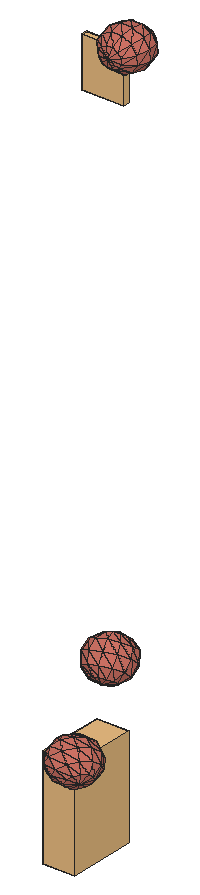
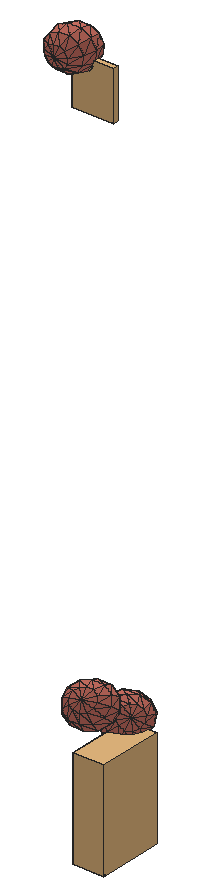
# SketchUp Ruby script. Lengths in inches.
U = 1.inch
M = Sketchup.active_model
def pt(a) = Geom::Point3d.new(a.map { |v| v * U })
def face(e, loops, mat)
  f = e.add_face(loops[0].map { |a| pt(a) })
  loops[1..].each { |l| e.add_face(l.map { |a| pt(a) }).erase! }
  f.material = f.back_material = mat if mat
  f
end
# faces: each face lists its corners as indices into pts; further lists are holes
def faces(e, pts, list, mat = nil) = list.each { |f| face(e, (f[0].is_a?(Array) ? f : [f]).map { |l| l.map { |i| pts[i] } }, mat) }
# xy, xz, yz: faces in a plane at the given z, y or x. An outline is a flat list of corners, or four numbers for a rectangle; further outlines are holes
def ring(l) = l.size == 4 ? [[l[0], l[1]], [l[2], l[1]], [l[2], l[3]], [l[0], l[3]]] : l.each_slice(2).to_a
def flat(e, list, mat, &to3) = list.each { |f| face(e, (f[0].is_a?(Array) ? f : [f]).map { |l| ring(l).map { |u, v| to3.(u, v) } }, mat) }
def xy(e, z, list, mat = nil) = flat(e, list, mat) { |x, y| [x, y, z] }
def xz(e, y, list, mat = nil) = flat(e, list, mat) { |x, z| [x, y, z] }
def yz(e, x, list, mat = nil) = flat(e, list, mat) { |y, z| [x, y, z] }
def lines(e, pts, list) = list.each { |a, b| e.add_line(pt(pts[a]), pt(pts[b])) }
# prism: a flat outline (further loops are holes) pulled along v
def prism(e, loops, v, mat = nil)
  f = face(e, loops, mat); d = Geom::Vector3d.new(v.map { |x| x * U })
  f.pushpull(f.normal.samedirection?(d) ? d.length : -d.length)
end
def box(e, o, s, mat = nil) = prism(e, [[o, [o[0] + s[0], o[1], o[2]], [o[0] + s[0], o[1] + s[1], o[2]], [o[0], o[1] + s[1], o[2]]]], [0, 0, s[2]], mat)
def at(x, y, z, deg = 0) = Geom::Transformation.translation(pt([x, y, z])) * Geom::Transformation.rotation(ORIGIN, Z_AXIS, deg.degrees)
def axes(o, x, y, z) = Geom::Transformation.new([*x, 0, *y, 0, *z, 0, *pt(o).to_a, 1])
def part(name) = M.definitions.add(name)
# library, detail: a bought-in or finely detailed component or shape, given as its bounding box
def library(name, o, s) = part(name).tap { |d| box(d.entities, o, s) }
def detail(e, o, s) = box(e.add_group.entities, o, s)
def put(e, d, t, mat = nil) = e.add_instance(d, t).tap { |i| i.material = mat if mat }
def group(e, t, mat = nil) = e.add_group.tap { |g| g.transformation = t; g.material = mat if mat }.entities
root = M.entities
M.materials.add("green").color = [174, 139, 102]
M.materials.add("vio").color = [206, 114, 100]
c1 = part("3DGeom~239_Defintion")
p = [[90.53,-63.37,-491.99],[67.74,-328.31,-318.83],[-81.52,-183.54,-449.92],[266.4,-189.55,-367.41],[200.76,100.79,-448.8],[-109.61,79.79,-484.74],
  [-45.97,174.5625,-459.8],[-208.9375,10.41,-460.45],[-280.37,201.57,-347.6],[-269.29,-227.52,-333.86],[-317.35,-14.98,-393.44],[-35.07,269.34,-392.33],
  [-149.08,-379.1,-184.82],[393.68,0,-317.54],[219.63,264.9375,-331.92],[-317.35,-14.98,-393.44],[-269.29,-227.52,-333.86],[-422.46,-183.54,-174.92],
  [-317.35,-14.98,-393.44],[-405.78,10.41,-301.68],[-405.78,10.41,-301.68],[-79.84,338.72,-300.39],[-79.84,338.72,-300.39],[219.63,264.9375,-331.92],
  [-35.07,269.34,-392.33],[266.4,-189.55,-367.41],[198.85,-385.11,-102.31],[67.74,-328.31,-318.83],[266.4,-189.55,-367.41],[370.9,-264.9375,-144.38],
  [393.68,0,-317.54],[370.9,-264.9375,-144.38],[266.4,-189.55,-367.41],[-450.55,79.79,-209.74],[-280.37,201.57,-347.6],[-439.65,174.5625,-142.26],
  [-280.37,201.57,-347.6],[-376.01,269.34,-117.33],[-280.37,201.57,-347.6],[-276.68,338.72,-141.62],[-280.37,201.57,-347.6],[-168.27,364.11,-208.62],
  [-276.68,338.72,-141.62],[-168.27,364.11,-208.62],[-280.37,201.57,-347.6],[-269.29,-227.52,-333.86],[-149.08,-379.1,-184.82],[-325.95,-328.31,-1.29],
  [-269.29,-227.52,-333.86],[415.48,189.55,-182.59],[142.09,385.11,-172.68],[415.48,189.55,-182.59],[219.63,264.9375,-331.92],[-79.84,338.72,-300.39],
  [219.63,264.9375,-331.92],[67.74,-328.31,-318.83],[11.08,-429.09,13.74],[-149.08,-379.1,-184.82],[67.74,-328.31,-318.83],[393.68,0,-317.54],
  [481.125,-100.79,-101.2],[370.9,-264.9375,-144.38],[415.48,189.55,-182.59],[393.68,0,-317.54],[-500,-63.37,-15.68],[-168.27,364.11,-208.62],
  [-79.84,338.72,-300.39],[-481.125,100.79,101.2],[-11.08,429.09,-13.74],[-168.27,364.11,-208.62],[-168.27,364.11,-208.62],[-149.08,-379.1,-184.82],
  [-142.09,-385.11,172.68],[-149.08,-379.1,-184.82],[-325.95,-328.31,-1.29],[415.48,189.55,-182.59],[500,63.37,15.68],[325.95,328.31,1.29],
  [415.48,189.55,-182.59],[325.95,328.31,1.29],[415.48,189.55,-182.59],[-415.48,-189.55,182.59],[276.68,-338.72,141.62],[376.01,-269.34,117.33],
  [376.01,-269.34,117.33],[370.9,-264.9375,-144.38],[-370.9,264.9375,144.38],[-370.9,264.9375,144.38],[-376.01,269.34,-117.33],[-198.85,385.11,102.31],
  [-376.01,269.34,-117.33],[-370.9,264.9375,144.38],[168.27,-364.11,208.62],[439.65,-174.5625,142.26],[376.01,-269.34,117.33],[-393.68,0,317.54],
  [149.08,379.1,184.82],[-325.95,-328.31,-1.29],[-219.63,-264.9375,331.93],[-325.95,-328.31,-1.29],[-219.63,-264.9375,331.93],[-415.48,-189.55,182.59],
  [325.95,328.31,1.29],[422.46,183.54,174.92],[149.08,379.1,184.82],[325.95,328.31,1.29],[79.84,-338.72,300.39],[450.55,-79.79,209.74],
  [-266.4,189.55,367.41],[-266.4,189.55,367.41],[-370.9,264.9375,144.38],[-67.74,328.31,318.83],[276.68,-338.72,141.62],[376.01,-269.34,117.33],
  [280.37,-201.57,347.6],[376.01,-269.34,117.33],[280.37,-201.57,347.6],[280.37,-201.57,347.6],[280.37,-201.57,347.6],[-266.4,189.55,367.41],
  [35.07,-269.34,392.33],[-219.63,-264.9375,331.93],[35.07,-269.34,392.33],[405.78,-10.41,301.68],[269.29,227.52,333.86],[149.08,379.1,184.82],
  [-415.48,-189.55,182.59],[-219.63,-264.9375,331.93],[-200.76,-100.78,448.8],[-415.48,-189.55,182.59],[-393.68,0,317.54],[-67.74,328.31,318.83],
  [269.29,227.52,333.86],[149.08,379.1,184.82],[79.84,-338.72,300.39],[168.27,-364.11,208.62],[280.37,-201.57,347.6],[280.37,-201.57,347.6],
  [35.07,-269.34,392.33],[79.84,-338.72,300.39],[280.37,-201.57,347.6],[405.78,-10.41,301.68],[317.35,14.98,393.44],[280.37,-201.57,347.6],
  [317.35,14.98,393.44],[-393.68,0,317.54],[-90.53,63.37,491.99],[-393.68,0,317.54],[-266.4,189.55,367.41],[-266.4,189.55,367.41],
  [81.52,183.54,449.92],[-67.74,328.31,318.83],[-67.74,328.31,318.83],[269.29,227.52,333.86],[45.97,-174.5625,459.8],[317.35,14.98,393.44],
  [269.29,227.52,333.86],[280.37,-201.57,347.6],[109.61,-79.79,484.74],[280.37,-201.57,347.6],[208.9375,-10.41,460.45],[280.37,-201.57,347.6],
  [317.35,14.98,393.44],[280.37,-201.57,347.6],[-266.4,189.55,367.41],[317.35,14.98,393.44]]
faces(c1.entities,p,[[0,1,2],[0,3,1],[4,3,0],[5,0,2],[6,0,5],[6,4,0],[5,2,7],[5,7,8],
  [6,5,8],[7,9,10],[7,2,9],[7,10,8],[11,4,6],[11,6,8],[2,12,9],[2,1,12],
  [4,13,3],[14,13,4],[11,14,4],[15,16,17],[18,17,19],[10,20,8],[21,11,8],[22,23,24],
  [25,26,27],[28,29,26],[30,31,32],[19,33,34],[33,35,36],[35,37,38],[37,39,40],[41,21,8],
  [42,43,44],[45,46,47],[48,47,17],[14,49,13],[50,51,52],[53,50,54],[55,56,57],[58,26,56],
  [59,60,61],[62,60,63],[19,17,64],[19,64,33],[65,50,66],[33,64,67],[33,67,35],[42,68,69],
  [70,68,50],[71,56,72],[73,72,74],[75,76,60],[77,76,78],[50,79,80],[17,47,81],[17,81,64],
  [68,79,50],[29,82,26],[29,83,82],[60,84,85],[35,67,86],[35,87,37],[88,89,42],[42,89,68],
  [90,91,89],[26,92,56],[26,82,92],[60,93,94],[76,93,60],[64,81,95],[64,95,67],[68,96,79],
  [89,96,68],[97,72,98],[99,100,101],[102,103,76],[104,103,105],[56,106,72],[56,92,106],[76,107,93],
  [103,107,76],[67,95,108],[67,109,110],[91,111,89],[89,111,96],[112,113,114],[115,93,116],[92,82,117],
  [93,107,118],[91,119,111],[72,120,121],[72,106,122],[103,123,107],[124,123,103],[125,124,103],[126,127,128],
  [129,128,130],[131,132,133],[134,135,136],[107,123,137],[138,139,140],[141,142,143],[124,144,123],[145,128,146],
  [147,146,148],[149,150,151],[152,150,153],[127,138,154],[127,154,128],[150,155,156],[154,138,157],[158,154,159],
  [160,158,161],[162,160,163],[164,146,150],[150,160,165],[128,154,158],[128,158,146],[146,160,150],[146,158,160]],"vio")
c2 = library("3DGeom~163_Defintion",[-333.59,-500,-156.82],[667.18,1000,313.64])
c3 = part("3DGeom~164_Defintion")
p = [[-316.7,-484.43,-156.82],[-330.53,-495.14,-131.21],[-331.78,-487.36,-147.01],[-300.37,-489.29,-150.82],[-330.53,-495.14,-131.21],[-316.7,-484.43,-156.82],
  [-300.37,-489.29,-150.82],[-316.7,-484.43,-156.82],[-307.47,-486.03,-155.8],[-316.7,-484.43,-156.82],[-331.78,-487.36,-147.01],[-325.6,-484.92,-153.6],
  [-299.12,-497.07,-135.02],[-330.53,-495.14,-131.21],[-300.37,-489.29,-150.82],[-299.12,-497.07,-135.02],[-300.37,-489.29,-150.82],[-297.3125,-493.33,-143.21],
  [-330.53,-495.14,-131.21],[-333.59,-491.1,-138.82],[-331.78,-487.36,-147.01],[-314.2,-500,-125.21],[-330.53,-495.14,-131.21],[-299.12,-497.07,-135.02],
  [-314.2,-500,-125.21],[-299.12,-497.07,-135.02],[-305.3,-499.51,-128.43],[-330.53,-495.14,-131.21],[-314.2,-500,-125.21],[-323.43,-498.4,-126.23],
  [306.85,495.99,152.28],[330.06,486.75,126.11],[323.43,491.02,121.57],[306.85,495.99,152.28],[323.43,491.02,121.57],[315.47,495.38,121.75],
  [306.85,495.99,152.28],[315.47,495.38,121.75],[308.3,498.67,126.61],[306.85,495.99,152.28],[333.59,483.72,134.16],[330.06,486.75,126.11],
  [306.85,495.99,152.28],[308.3,498.67,126.61],[303.86,500,134.83],[306.85,495.99,152.28],[333.05,482.74,143.56],[333.59,483.72,134.16],
  [306.85,495.99,152.28],[303.86,500,134.83],[303.33,499.02,144.23],[306.85,495.99,152.28],[328.61,484.07,151.78],[333.05,482.74,143.56],
  [306.85,495.99,152.28],[321.44,487.36,156.64],[328.61,484.07,151.78],[306.85,495.99,152.28],[313.48,491.72,156.82],[321.44,487.36,156.64]]
faces(c3.entities,p,[[0,1,2],[3,4,5],[6,7,8],[9,10,11],[12,13,14],[15,16,17],[18,19,20],[21,22,23],
  [24,25,26],[27,28,29],[30,31,32],[33,34,35],[36,37,38],[39,40,41],[42,43,44],[45,46,47],
  [48,49,50],[51,52,53],[54,55,56],[57,58,59]],"green")
c4 = part("3DGeom~249_Defintion")
p = [[-255.5,94.92,-415.28],[-6.35,103.625,-485.08],[-12.59,-116.1,-481.02],[239.09,-105.72,-421.38],[244.5,84.5625,-424.9],[1.59,295.58,-359.16],
  [-248.62,261.16,-306.23],[-255.5,94.92,-415.28],[-248.62,261.16,-306.23],[-260.91,-95.36,-411.76],[-15.46,-304.71,-348.07],[236.61,-269.07,-306.25],
  [-255.5,94.92,-415.28],[-260.91,-95.36,-411.76],[426.72,-67.02,-248.84],[429.84,42.84,-250.87],[426.72,-67.02,-248.84],[251.38,250.8,-315.85],
  [429.84,42.84,-250.87],[244.5,84.5625,-424.9],[251.38,250.8,-315.85],[239.09,-105.72,-421.38],[425.28,-161.33,-182.37],[236.61,-269.07,-306.25],
  [239.09,-105.72,-421.38],[426.72,-67.02,-248.84],[-436.1875,60.78,-234.21],[-255.5,94.92,-415.28],[-260.91,-95.36,-411.76],[-432.22,156.76,-171.25],
  [-248.62,261.16,-306.23],[-260.91,-95.36,-411.76],[-263.39,-258.71,-296.63],[-439.31,-49.07,-232.18],[-263.39,-258.71,-296.63],[9.11,408.34,-137.01],
  [251.38,250.8,-315.85],[1.59,295.58,-359.16],[-242.11,358.81,-113.84],[1.59,295.58,-359.16],[-248.62,261.16,-306.23],[-242.11,358.81,-113.84],
  [1.59,295.58,-359.16],[-263.39,-258.71,-296.63],[-15.46,-304.71,-348.07],[-14.18,-411.68,-121.86],[-15.46,-304.71,-348.07],[237.72,-361.7,-110.34],
  [-15.46,-304.71,-348.07],[236.61,-269.07,-306.25],[251.38,250.8,-315.85],[433.81,138.82,-187.91],[429.84,42.84,-250.87],[257.89,348.45,-123.46],
  [251.38,250.8,-315.85],[257.89,348.45,-123.46],[251.38,250.8,-315.85],[236.61,-269.07,-306.25],[425.92,-214.8125,-69.26],[237.72,-361.7,-110.34],
  [236.61,-269.07,-306.25],[-428.46,213.14,-60.17],[-242.11,358.81,-113.84],[-263.39,-258.71,-296.63],[-262.28,-351.34,-100.72],[-440.74,-143.38,-165.7],
  [-262.28,-351.34,-100.72],[429.84,42.84,-250.87],[500,-10.36,-9.62],[429.84,42.84,-250.87],[-500,10.36,9.62],[437.57,195.19,-76.83],
  [257.89,348.45,-123.46],[-440.1,-196.87,-52.6],[14.18,411.68,121.86],[-237.72,361.7,110.34],[-242.11,358.81,-113.84],[-237.72,361.7,110.34],
  [262.28,351.34,100.72],[257.89,348.45,-123.46],[262.28,351.34,100.72],[-262.28,-351.34,-100.72],[-9.11,-408.34,137.01],[242.11,-358.81,113.84],
  [-425.92,214.8125,69.26],[-237.72,361.7,110.34],[237.72,-361.7,-110.34],[428.46,-213.14,60.17],[237.72,-361.7,-110.34],[242.11,-358.81,113.84],
  [-262.28,-351.34,-100.72],[-257.89,-348.45,123.46],[-257.89,-348.45,123.46],[440.1,196.87,52.6],[262.28,351.34,100.72],[-437.57,-195.19,76.83],
  [432.22,-156.76,171.25],[436.1875,-60.78,234.21],[439.31,49.07,232.18],[440.74,143.38,165.7],[-433.81,-138.82,187.91],[-429.84,-42.84,250.87],
  [-426.72,67.02,248.84],[-425.28,161.33,182.37],[263.39,258.71,296.63],[263.39,258.71,296.63],[262.28,351.34,100.72],[242.11,-358.81,113.84],
  [-251.38,-250.8,315.85],[15.46,304.71,348.07],[263.39,258.71,296.63],[-236.61,269.07,306.25],[-236.61,269.07,306.25],[-237.72,361.7,110.34],
  [248.62,-261.16,306.23],[242.11,-358.81,113.84],[248.62,-261.16,306.23],[-236.61,269.07,306.25],[-257.89,-348.45,123.46],[-1.59,-295.58,359.16],
  [-257.89,-348.45,123.46],[-1.59,-295.58,359.16],[-251.38,-250.8,315.85],[248.62,-261.16,306.23],[-1.59,-295.58,359.16],[260.91,95.36,411.76],
  [260.91,95.36,411.76],[263.39,258.71,296.63],[248.62,-261.16,306.23],[-244.5,-84.5625,424.9],[-244.5,-84.5625,424.9],[255.5,-94.92,415.28],
  [255.5,-94.92,415.28],[260.91,95.36,411.76],[248.62,-261.16,306.23],[255.5,-94.92,415.28],[-429.84,-42.84,250.87],[-239.09,105.73,421.38],
  [-426.72,67.02,248.84],[-239.09,105.73,421.38],[-429.84,-42.84,250.87],[-244.5,-84.5625,424.9],[-239.09,105.73,421.38],[12.59,116.1,481.02],
  [260.91,95.36,411.76],[263.39,258.71,296.63],[263.39,258.71,296.63],[15.46,304.71,348.07],[-1.59,-295.58,359.16],[248.62,-261.16,306.23],
  [255.5,-94.92,415.28],[-239.09,105.73,421.38],[15.46,304.71,348.07],[-236.61,269.07,306.25],[-251.38,-250.8,315.85],[6.35,-103.625,485.08],
  [-251.38,-250.8,315.85],[-239.09,105.73,421.38],[15.46,304.71,348.07],[-239.09,105.73,421.38]]
faces(c4.entities,p,[[0,1,2],[1,3,2],[1,4,3],[5,4,1],[6,1,7],[8,5,1],[9,2,10],[2,11,10],
  [2,3,11],[12,2,13],[4,14,3],[4,15,16],[17,18,19],[5,20,4],[21,22,23],[24,25,22],
  [26,27,28],[29,27,26],[29,30,27],[31,10,32],[33,28,34],[26,28,33],[35,36,37],[38,39,40],
  [41,35,42],[43,44,45],[46,47,45],[48,49,47],[50,51,52],[53,51,54],[35,55,56],[57,58,59],
  [60,22,58],[61,30,29],[61,62,30],[63,45,64],[65,34,66],[33,34,65],[25,67,68],[69,51,68],
  [22,25,68],[26,33,70],[29,26,70],[33,65,70],[51,71,68],[72,71,51],[58,22,68],[61,29,70],
  [65,66,73],[65,73,70],[74,55,35],[75,35,76],[77,74,35],[78,71,79],[74,80,55],[81,45,82],
  [45,47,83],[45,83,82],[84,62,61],[84,85,62],[86,58,87],[88,87,89],[90,82,91],[73,66,92],
  [71,93,68],[94,93,71],[87,58,68],[84,61,70],[73,92,95],[73,95,70],[96,87,68],[97,96,68],
  [98,97,68],[99,98,68],[93,99,68],[95,100,70],[100,101,70],[101,102,70],[103,84,70],[102,103,70],
  [104,99,93],[105,93,106],[107,87,96],[103,85,84],[95,92,108],[95,108,100],[109,110,80],[109,80,74],
  [103,111,85],[112,74,113],[82,83,114],[115,96,116],[117,109,74],[118,82,119],[120,121,122],[82,123,124],
  [125,98,99],[126,99,127],[128,96,97],[102,111,103],[100,108,129],[100,130,101],[131,97,98],[132,98,133],
  [134,97,135],[136,137,138],[102,139,111],[140,141,142],[143,144,145],[143,146,147],[148,149,150],[151,152,153],
  [154,148,155],[156,155,141],[157,143,158],[148,150,155],[155,150,144],[155,144,143],[141,143,159],[141,155,143]],"vio")
c5 = library("3DGeom~183_Defintion",[-58.28,-500,-420.6],[116.56,1000,841.2])
c6 = part("3DGeom~184_Defintion")
p = [[-21.41,-458.84,-420.6],[-21.53,-500,-365.15],[-53.32,-468.47,-406.125],[10.44,-469.79,-407.35],[-21.53,-500,-365.15],[10.44,-469.79,-407.35],
  [-3.01,-461.98,-417.24],[-53.32,-468.47,-406.125],[-39.83,-461.21,-416.53],[10.38,-490.37,-379.625],[-21.53,-500,-365.15],[10.44,-469.79,-407.35],
  [10.38,-490.37,-379.625],[10.44,-469.79,-407.35],[15.34,-480.18,-393.58],[-53.32,-468.47,-406.125],[-21.53,-500,-365.15],[-53.38,-489.05,-378.4],
  [-53.32,-468.47,-406.125],[-53.38,-489.05,-378.4],[-58.28,-478.66,-392.17],[-21.53,-500,-365.15],[10.38,-490.37,-379.625],[-3.11,-497.625,-369.22],
  [-21.53,-500,-365.15],[-39.93,-496.86,-368.51],[-53.38,-489.05,-378.4],[21.98,487.39,420.6],[20.96,500,348.46],[2.62,499.54,353.65],
  [21.98,487.39,420.6],[39.43,498.77,352.9375],[20.96,500,348.46],[21.98,487.39,420.6],[53.09,496.1875,365.88],[39.43,498.77,352.9375],
  [21.98,487.39,420.6],[2.62,499.54,353.65],[-10.67,497.51,367.11],[21.98,487.39,420.6],[58.28,492.93,383.82],[53.09,496.1875,365.88],
  [21.98,487.39,420.6],[-10.67,497.51,367.11],[-15.34,494.46,385.24],[21.98,487.39,420.6],[53.61,489.88,401.95],[58.28,492.93,383.82],
  [21.98,487.39,420.6],[-15.34,494.46,385.24],[-10.15,491.2,403.18],[21.98,487.39,420.6],[40.32,487.85,415.41],[53.61,489.88,401.95],
  [21.98,487.39,420.6],[-10.15,491.2,403.18],[3.51,488.61,416.12]]
faces(c6.entities,p,[[0,1,2],[3,4,0],[5,0,6],[0,7,8],[9,10,11],[12,13,14],[15,16,17],[18,19,20],
  [21,22,23],[24,25,26],[27,28,29],[30,31,32],[33,34,35],[36,37,38],[39,40,41],[42,43,44],
  [45,46,47],[48,49,50],[51,52,53],[54,55,56]],"green")
c7 = part("3DGeom~215_Defintion")
p = [[153.1,0,-493.4375],[146.71,-288.7,-360.18],[-37.25,-159.0625,-480.02],[311.55,-150.94,-371.8],[-46.38,150.94,-482.85],[302.41,159.0625,-374.64],
  [82.93,288.7,-379.97],[-211.22,13.19,-471.24],[-233.43,261.44,-342.89],[-158.77,340.98,-283.49],[-233.43,261.44,-342.89],[-158.77,340.98,-283.49],
  [-9.49,-389.54,-237.18],[-217.61,-275.51,-337.98],[-9.49,-389.54,-237.18],[-217.61,-275.51,-337.98],[-217.61,-275.51,-337.98],[-367.42,-87.65,-348.23],
  [-328.6,181.91,-336.18],[-367.42,-87.65,-348.23],[-233.43,261.44,-342.89],[-328.6,181.91,-336.18],[142.07,389.54,-190.15],[-124.625,399.2,-173.9],
  [82.93,288.7,-379.97],[-158.77,340.98,-283.49],[142.07,389.54,-190.15],[82.93,288.7,-379.97],[440.86,-13.19,-268.92],[370.7,275.51,-155.45],
  [440.86,-13.19,-268.92],[302.41,159.0625,-374.64],[142.07,389.54,-190.15],[370.7,275.51,-155.45],[311.55,-150.94,-371.8],[291.35,-340.98,-143.84],
  [146.71,-288.7,-360.18],[311.55,-150.94,-371.8],[386.52,-261.44,-150.55],[291.35,-340.98,-143.84],[440.86,-13.19,-268.92],[311.55,-150.94,-371.8],
  [146.71,-288.7,-360.18],[201.17,-399.2,-72.82],[-9.49,-389.54,-237.18],[146.71,-288.7,-360.18],[291.35,-340.98,-143.84],[-367.42,-87.65,-348.23],
  [-339.66,-318.125,-105.38],[-473.12,-124.56,-146.79],[-217.61,-275.51,-337.98],[-418.78,123.69,-265.17],[-328.6,181.91,-336.18],[-367.42,-87.65,-348.23],
  [-418.78,123.69,-265.17],[-233.43,261.44,-342.89],[-328.6,181.91,-336.18],[-357.93,301.89,-111.05],[-233.43,261.44,-342.89],[-357.93,301.89,-111.05],
  [-217.61,-275.51,-337.98],[-115.19,-426.45,-35.74],[-339.66,-318.125,-105.38],[-217.61,-275.51,-337.98],[-357.93,301.89,-111.05],[440.86,-13.19,-268.92],
  [461.18,-181.91,-91.15],[500,87.65,-79.1],[440.86,-13.19,-268.92],[370.7,275.51,-155.45],[440.86,-13.19,-268.92],[-479.8,102.38,-148.87],
  [140.14,-420.51,43.48],[115.19,426.45,35.74],[370.7,275.51,-155.45],[-140.14,420.51,-43.48],[-357.93,301.89,-111.05],[339.66,318.125,105.38],
  [370.7,275.51,-155.45],[339.66,318.125,105.38],[370.7,275.51,-155.45],[291.35,-340.98,-143.84],[357.93,-301.89,111.05],[357.93,-301.89,111.05],
  [-500,-87.65,79.1],[-495.32,123.69,-18.45],[-370.7,-275.51,155.45],[357.93,-301.89,111.05],[-461.18,181.91,91.15],[-386.52,261.44,150.55],
  [-291.35,340.98,143.84],[-201.17,399.2,72.82],[-357.93,301.89,-111.05],[-291.35,340.98,143.84],[-357.93,301.89,-111.05],[-339.66,-318.125,-105.38],
  [-142.07,-389.54,190.15],[-339.66,-318.125,-105.38],[-142.07,-389.54,190.15],[-370.7,-275.51,155.45],[495.32,-123.69,18.45],[357.93,-301.89,111.05],
  [473.12,124.56,146.79],[339.66,318.125,105.38],[124.625,-399.2,173.9],[-142.07,-389.54,190.15],[-440.86,13.19,268.92],[479.8,-102.38,148.86],
  [357.93,-301.89,111.05],[9.49,389.54,237.18],[-302.41,-159.0625,374.64],[-302.41,-159.0625,374.64],[-311.55,150.94,371.8],[217.61,275.51,337.98],
  [339.66,318.125,105.38],[217.61,275.51,337.98],[158.77,-340.98,283.49],[233.43,-261.44,342.89],[158.77,-340.98,283.49],[328.6,-181.91,336.18],
  [233.43,-261.44,342.89],[357.93,-301.89,111.05],[418.78,-123.69,265.16],[328.6,-181.91,336.18],[357.93,-301.89,111.05],[357.93,-301.89,111.05],
  [-146.71,288.7,360.18],[-291.35,340.98,143.84],[-146.71,288.7,360.18],[367.42,87.65,348.23],[217.61,275.51,337.98],[-146.71,288.7,360.18],
  [-370.7,-275.51,155.45],[-142.07,-389.54,190.15],[-82.93,-288.7,379.97],[-370.7,-275.51,155.45],[-302.41,-159.0625,374.64],[-142.07,-389.54,190.15],
  [158.77,-340.98,283.49],[-142.07,-389.54,190.15],[158.77,-340.98,283.49],[-82.93,-288.7,379.97],[-146.71,288.7,360.18],[217.61,275.51,337.98],
  [9.49,389.54,237.18],[211.22,-13.19,471.24],[328.6,-181.91,336.18],[418.78,-123.69,265.16],[418.78,-123.69,265.16],[367.42,87.65,348.23],
  [-440.86,13.19,268.92],[-153.09,0,493.4375],[-440.86,13.19,268.92],[-311.55,150.94,371.8],[158.77,-340.98,283.49],[233.43,-261.44,342.89],
  [46.38,-150.94,482.85],[37.25,159.0625,480.02],[367.42,87.65,348.23],[217.61,275.51,337.98],[-146.71,288.7,360.18],[217.61,275.51,337.98],
  [367.42,87.65,348.23],[-311.55,150.94,371.8],[-146.71,288.7,360.18],[-311.55,150.94,371.8]]
faces(c7.entities,p,[[0,1,2],[0,3,1],[4,0,2],[5,3,0],[6,0,4],[6,5,0],[4,2,7],[8,4,7],
  [9,4,10],[11,6,4],[2,12,13],[2,1,14],[7,2,15],[7,16,17],[18,7,19],[20,7,21],
  [22,5,6],[23,24,25],[23,26,27],[5,28,3],[29,30,31],[32,33,5],[34,35,36],[37,38,39],
  [40,38,41],[42,43,44],[45,46,43],[47,48,49],[47,50,48],[51,47,49],[52,53,54],[55,56,57],
  [25,58,59],[60,61,62],[63,44,61],[56,51,57],[23,25,64],[65,66,38],[67,66,68],[69,67,70],
  [51,49,71],[51,71,57],[44,72,61],[44,43,72],[73,74,26],[75,73,26],[75,26,23],[75,23,76],
  [77,67,78],[73,79,80],[81,38,82],[38,66,83],[71,49,84],[71,84,85],[71,85,57],[49,48,86],
  [49,86,84],[43,46,87],[85,88,57],[88,89,57],[89,90,57],[91,75,92],[93,91,94],[95,61,96],
  [97,98,99],[66,100,101],[67,100,66],[102,100,67],[103,102,67],[72,43,87],[91,73,75],[61,104,105],
  [61,72,104],[85,84,106],[85,106,88],[100,107,108],[102,107,100],[109,79,73],[91,109,73],[104,72,87],
  [93,109,91],[84,86,110],[84,111,106],[88,106,112],[88,112,89],[113,102,114],[109,115,79],[116,104,87],
  [117,118,87],[119,120,121],[122,123,124],[107,122,125],[89,126,127],[93,128,109],[129,107,102],[130,129,102],
  [129,122,107],[89,112,131],[132,133,134],[135,134,136],[137,104,138],[139,140,141],[142,143,144],[145,146,147],
  [145,148,149],[150,136,151],[152,151,153],[134,154,155],[156,155,146],[156,146,145],[157,158,159],[160,157,161],
  [134,155,156],[157,145,162],[163,157,164],[165,151,157],[136,134,156],[136,156,151],[151,156,145],[151,145,157]],"vio")
g1 = group(root,at(15.3125,38.42,26.21))
put(g1,c1,axes([-1.05,-1.04,10.17],[0,0.00039,0],[0,0,-0.00039],[-0.00039,0,0]),"vio")
g2 = group(root,at(15.3125,38.42,26.21))
put(g2,c2,axes([-1.18,-0.76,9.74],[0,0.00081,0],[0,0,-0.00081],[-0.00081,0,0]),"green")
put(g2,c3,axes([-1.18,-0.76,9.74],[0,0.00081,0],[0,0,-0.00081],[-0.00081,0,0]),"green")
g3 = group(root,at(15.3125,38.42,26.21))
put(g3,c4,axes([-0.95,-0.63,15.18],[0,0.00039,0],[0,0,-0.00039],[-0.00039,0,0]),"vio")
g4 = group(root,at(15.3125,38.42,26.21))
put(g4,c5,axes([-1.13,-0.625,14.96],[0,0.0004,0],[0,0,-0.0004],[-0.0004,0,0]),"green")
put(g4,c6,axes([-1.13,-0.625,14.96],[0,0.0004,0],[0,0,-0.0004],[-0.0004,0,0]),"green")
g5 = group(root,at(15.3125,38.42,26.21))
put(g5,c7,axes([-1.24,-0.44,10.58],[0,0.00038,0],[0,0,-0.00038],[-0.00038,0,0]),"vio")
